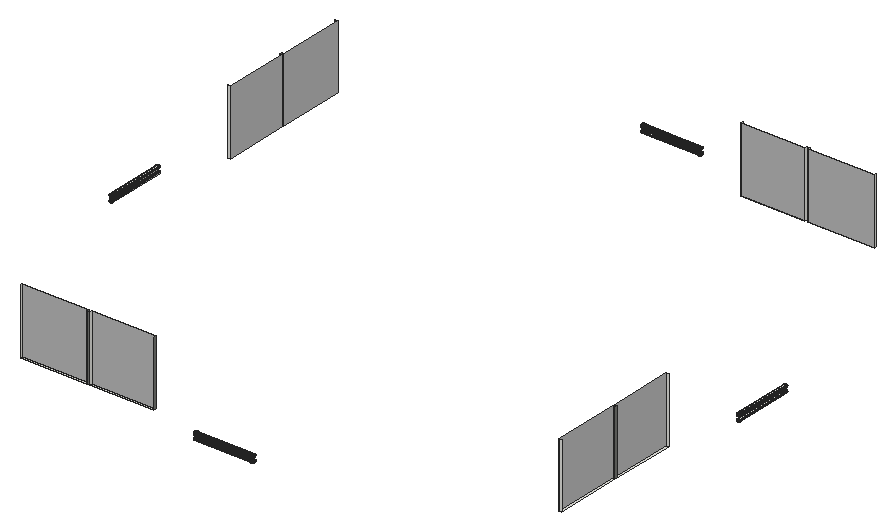
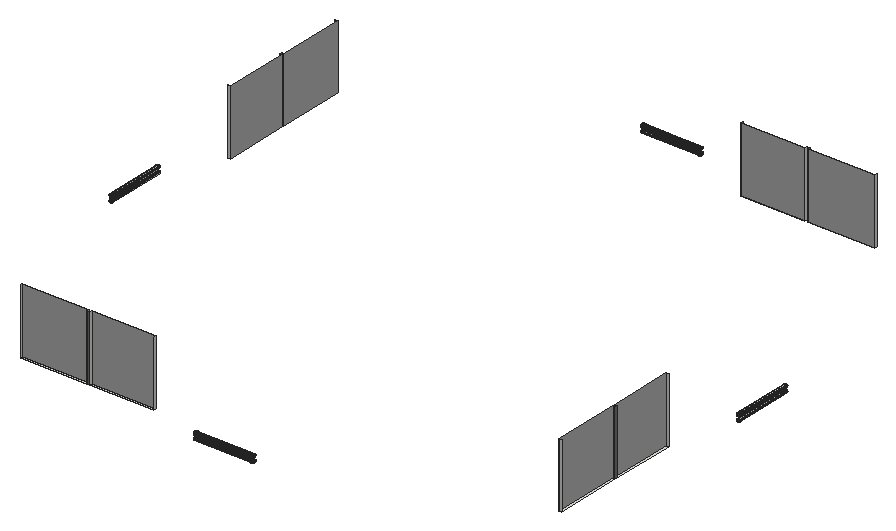
# SketchUp Ruby script. Lengths in inches.
U = 1.inch
M = Sketchup.active_model
def pt(a) = Geom::Point3d.new(a.map { |v| v * U })
def face(e, loops, mat)
  f = e.add_face(loops[0].map { |a| pt(a) })
  loops[1..].each { |l| e.add_face(l.map { |a| pt(a) }).erase! }
  f.material = f.back_material = mat if mat
  f
end
# faces: each face lists its corners as indices into pts; further lists are holes
def faces(e, pts, list, mat = nil) = list.each { |f| face(e, (f[0].is_a?(Array) ? f : [f]).map { |l| l.map { |i| pts[i] } }, mat) }
# xy, xz, yz: faces in a plane at the given z, y or x. An outline is a flat list of corners, or four numbers for a rectangle; further outlines are holes
def ring(l) = l.size == 4 ? [[l[0], l[1]], [l[2], l[1]], [l[2], l[3]], [l[0], l[3]]] : l.each_slice(2).to_a
def flat(e, list, mat, &to3) = list.each { |f| face(e, (f[0].is_a?(Array) ? f : [f]).map { |l| ring(l).map { |u, v| to3.(u, v) } }, mat) }
def xy(e, z, list, mat = nil) = flat(e, list, mat) { |x, y| [x, y, z] }
def xz(e, y, list, mat = nil) = flat(e, list, mat) { |x, z| [x, y, z] }
def yz(e, x, list, mat = nil) = flat(e, list, mat) { |y, z| [x, y, z] }
def lines(e, pts, list) = list.each { |a, b| e.add_line(pt(pts[a]), pt(pts[b])) }
# prism: a flat outline (further loops are holes) pulled along v
def prism(e, loops, v, mat = nil)
  f = face(e, loops, mat); d = Geom::Vector3d.new(v.map { |x| x * U })
  f.pushpull(f.normal.samedirection?(d) ? d.length : -d.length)
end
def box(e, o, s, mat = nil) = prism(e, [[o, [o[0] + s[0], o[1], o[2]], [o[0] + s[0], o[1] + s[1], o[2]], [o[0], o[1] + s[1], o[2]]]], [0, 0, s[2]], mat)
def at(x, y, z, deg = 0) = Geom::Transformation.translation(pt([x, y, z])) * Geom::Transformation.rotation(ORIGIN, Z_AXIS, deg.degrees)
def axes(o, x, y, z) = Geom::Transformation.new([*x, 0, *y, 0, *z, 0, *pt(o).to_a, 1])
def part(name) = M.definitions.add(name)
# library, detail: a bought-in or finely detailed component or shape, given as its bounding box
def library(name, o, s) = part(name).tap { |d| box(d.entities, o, s) }
def detail(e, o, s) = box(e.add_group.entities, o, s)
def put(e, d, t, mat = nil) = e.add_instance(d, t).tap { |i| i.material = mat if mat }
def group(e, t, mat = nil) = e.add_group.tap { |g| g.transformation = t; g.material = mat if mat }.entities
root = M.entities
M.materials.add("[Metal Seamed]").color = [118, 119, 115]
M.materials.add("[Mirror 01]").color = [185, 185, 185]
xy(root,899.76,[[312.65,102.8125,473.9375,108.8125],[479.9375,102.8125,635.22,108.8125],[1476,277.47,1482,438.75],[1476,444.75,1482,600.03],[138,949.59,144,1104.875],
  [138,1110.875,144,1272.16],[984.78,1440.8125,1140.0625,1446.8125],[1146.0625,1440.8125,1307.35,1446.8125]])
xz(root,102.8125,[[473.9375,899.76,479.9375,1056.625]],"[Metal Seamed]")
xz(root,108.8125,[[312.65,899.76,473.9375,1056.625],[479.9375,899.76,635.22,1056.625]],"[Mirror 01]")
xz(root,277.47,[[1476,899.76,1482,1056.625]])
xz(root,438.75,[[1476,899.76,1482,1056.625]])
xz(root,444.75,[[1476,899.76,1482,1056.625]])
xz(root,600.03,[[1476,899.76,1482,1056.625]])
xz(root,949.59,[[138,899.76,144,1056.625]])
xz(root,1104.875,[[138,899.76,144,1056.625]])
xz(root,1110.875,[[138,899.76,144,1056.625]])
xz(root,1272.16,[[138,899.76,144,1056.625]])
xz(root,1440.8125,[[984.78,899.76,1140.0625,1056.625],[1146.0625,899.76,1307.35,1056.625]],"[Mirror 01]")
xz(root,1446.8125,[[1140.0625,899.76,1146.0625,1056.625]],"[Metal Seamed]")
yz(root,138,[[1104.875,899.76,1110.875,1056.625]],"[Metal Seamed]")
yz(root,144,[[949.59,899.76,1104.875,1056.625],[1110.875,899.76,1272.16,1056.625]],"[Mirror 01]")
yz(root,312.65,[[102.8125,899.76,108.8125,1056.625]])
yz(root,473.9375,[[102.8125,899.76,108.8125,1056.625]],"[Metal Seamed]")
yz(root,479.9375,[[102.8125,899.76,108.8125,1056.625]])
yz(root,635.22,[[102.8125,899.76,108.8125,1056.625]],"[Metal Seamed]")
yz(root,984.78,[[1440.8125,899.76,1446.8125,1056.625]])
yz(root,1140.0625,[[1440.8125,899.76,1446.8125,1056.625]])
yz(root,1146.0625,[[1440.8125,899.76,1446.8125,1056.625]])
yz(root,1307.35,[[1440.8125,899.76,1446.8125,1056.625]])
yz(root,1476,[[277.47,899.76,438.75,1056.625],[444.75,899.76,600.03,1056.625]],"[Mirror 01]")
yz(root,1482,[[438.75,899.76,444.75,1056.625]],"[Metal Seamed]")
p = [[922.01,48.34,909.02],[922.01,47.38,909.14],[778.64,47.38,909.14],[778.64,48.34,909.02],[922.01,49.29,909.14],[778.64,49.29,909.14],
  [83.53,662.8,909.02],[82.57,662.8,909.14],[82.57,806.17,909.14],[83.53,806.17,909.02],[84.48,662.8,909.14],[84.48,806.17,909.14],
  [1535.52,886.83,909.14],[1536.47,886.83,909.02],[1536.47,743.45,909.02],[1535.52,743.45,909.14],[1537.43,886.83,909.14],[1537.43,743.45,909.14],
  [697.99,1500.33,909.14],[697.99,1501.28,909.02],[841.36,1501.28,909.02],[841.36,1500.33,909.14],[697.99,1502.24,909.14],[841.36,1502.24,909.14],
  [922.01,46.5,909.51],[778.64,46.5,909.51],[922.01,50.18,909.51],[778.64,50.18,909.51],[81.68,662.8,909.51],[81.68,806.17,909.51],
  [85.37,662.8,909.51],[85.37,806.17,909.51],[1534.63,886.83,909.51],[1534.63,743.45,909.51],[1538.32,886.83,909.51],[1538.32,743.45,909.51],
  [697.99,1499.44,909.51],[841.36,1499.44,909.51],[697.99,1503.13,909.51],[841.36,1503.13,909.51],[922.01,45.73,910.1],[778.64,45.73,910.1],
  [922.01,50.95,910.1],[778.64,50.95,910.1],[80.92,662.8,910.1],[80.92,806.17,910.1],[86.13,662.8,910.1],[86.13,806.17,910.1],
  [1533.87,886.83,910.1],[1533.87,743.45,910.1],[1539.08,886.83,910.1],[1539.08,743.45,910.1],[697.99,1498.68,910.1],[841.36,1498.68,910.1],
  [697.99,1503.89,910.1],[841.36,1503.89,910.1],[922.01,45.15,910.86],[778.64,45.15,910.86],[922.01,51.53,910.86],[778.64,51.53,910.86],
  [80.33,662.8,910.86],[80.33,806.17,910.86],[86.72,662.8,910.86],[86.72,806.17,910.86],[1533.28,886.83,910.86],[1533.28,743.45,910.86],
  [1539.67,886.83,910.86],[1539.67,743.45,910.86],[697.99,1498.09,910.86],[841.36,1498.09,910.86],[697.99,1504.48,910.86],[841.36,1504.48,910.86],
  [922.01,44.78,911.75],[778.64,44.78,911.75],[922.01,51.9,911.75],[778.64,51.9,911.75],[79.97,662.8,911.75],[79.97,806.17,911.75],
  [87.09,662.8,911.75],[87.09,806.17,911.75],[1532.91,886.83,911.75],[1532.91,743.45,911.75],[1540.03,886.83,911.75],[1540.03,743.45,911.75],
  [697.99,1497.72,911.75],[841.36,1497.72,911.75],[697.99,1504.85,911.75],[841.36,1504.85,911.75],[922.01,44.65,912.7],[778.64,44.65,912.7],
  [922.01,52.03,912.7],[778.64,52.03,912.7],[79.84,662.8,912.7],[79.84,806.17,912.7],[87.21,662.8,912.7],[87.21,806.17,912.7],
  [1532.79,886.83,912.7],[1532.79,743.45,912.7],[1540.16,886.83,912.7],[1540.16,743.45,912.7],[697.99,1497.6,912.7],[841.36,1497.6,912.7],
  [697.99,1504.97,912.7],[841.36,1504.97,912.7],[922.01,44.78,913.66],[778.64,44.78,913.66],[922.01,51.9,913.66],[778.64,51.9,913.66],
  [79.97,662.8,913.66],[79.97,806.17,913.66],[87.09,662.8,913.66],[87.09,806.17,913.66],[1532.91,886.83,913.66],[1532.91,743.45,913.66],
  [1540.03,886.83,913.66],[1540.03,743.45,913.66],[697.99,1497.72,913.66],[841.36,1497.72,913.66],[697.99,1504.85,913.66],[841.36,1504.85,913.66],
  [922.01,45.15,914.55],[778.64,45.15,914.55],[922.01,51.53,914.55],[778.64,51.53,914.55],[80.33,662.8,914.55],[80.33,806.17,914.55],
  [86.72,662.8,914.55],[86.72,806.17,914.55],[1533.28,886.83,914.55],[1533.28,743.45,914.55],[1539.67,886.83,914.55],[1539.67,743.45,914.55],
  [697.99,1498.09,914.55],[841.36,1498.09,914.55],[697.99,1504.48,914.55],[841.36,1504.48,914.55],[922.01,45.73,915.3125],[778.64,45.73,915.3125],
  [922.01,50.95,915.3125],[778.64,50.95,915.3125],[80.92,662.8,915.3125],[80.92,806.17,915.3125],[86.13,662.8,915.3125],[86.13,806.17,915.3125],
  [1533.87,886.83,915.3125],[1533.87,743.45,915.3125],[1539.08,886.83,915.3125],[1539.08,743.45,915.3125],[697.99,1498.68,915.3125],[841.36,1498.68,915.3125],
  [697.99,1503.89,915.3125],[841.36,1503.89,915.3125],[922.01,46.5,915.9],[778.64,46.5,915.9],[922.01,50.18,915.9],[778.64,50.18,915.9],
  [81.68,662.8,915.9],[81.68,806.17,915.9],[85.37,662.8,915.9],[85.37,806.17,915.9],[1534.63,886.83,915.9],[1534.63,743.45,915.9],
  [1538.32,886.83,915.9],[1538.32,743.45,915.9],[697.99,1499.44,915.9],[841.36,1499.44,915.9],[697.99,1503.13,915.9],[841.36,1503.13,915.9],
  [922.01,47.38,916.27],[778.64,47.38,916.27],[922.01,49.29,916.27],[778.64,49.29,916.27],[82.57,662.8,916.27],[82.57,806.17,916.27],
  [84.48,662.8,916.27],[84.48,806.17,916.27],[1535.52,886.83,916.27],[1535.52,743.45,916.27],[1537.43,886.83,916.27],[1537.43,743.45,916.27],
  [697.99,1500.33,916.27],[841.36,1500.33,916.27],[697.99,1502.24,916.27],[841.36,1502.24,916.27],[922.01,48.34,916.39],[778.64,48.34,916.39],
  [83.53,662.8,916.39],[83.53,806.17,916.39],[1536.47,886.83,916.39],[1536.47,743.45,916.39],[697.99,1501.28,916.39],[841.36,1501.28,916.39],
  [922.01,48.34,921.02],[922.01,47.38,921.14],[778.64,47.38,921.14],[778.64,48.34,921.02],[922.01,49.29,921.14],[778.64,49.29,921.14],
  [83.53,662.8,921.02],[82.57,662.8,921.14],[82.57,806.17,921.14],[83.53,806.17,921.02],[84.48,662.8,921.14],[84.48,806.17,921.14],
  [1535.52,886.83,921.14],[1536.47,886.83,921.02],[1536.47,743.45,921.02],[1535.52,743.45,921.14],[1537.43,886.83,921.14],[1537.43,743.45,921.14],
  [697.99,1500.33,921.14],[697.99,1501.28,921.02],[841.36,1501.28,921.02],[841.36,1500.33,921.14],[697.99,1502.24,921.14],[841.36,1502.24,921.14],
  [922.01,46.5,921.51],[778.64,46.5,921.51],[922.01,50.18,921.51],[778.64,50.18,921.51],[81.68,662.8,921.51],[81.68,806.17,921.51],
  [85.37,662.8,921.51],[85.37,806.17,921.51],[1534.63,886.83,921.51],[1534.63,743.45,921.51],[1538.32,886.83,921.51],[1538.32,743.45,921.51],
  [697.99,1499.44,921.51],[841.36,1499.44,921.51],[697.99,1503.13,921.51],[841.36,1503.13,921.51],[922.01,45.73,922.1],[778.64,45.73,922.1],
  [922.01,50.95,922.1],[778.64,50.95,922.1],[80.92,662.8,922.1],[80.92,806.17,922.1],[86.13,662.8,922.1],[86.13,806.17,922.1],
  [1533.87,886.83,922.1],[1533.87,743.45,922.1],[1539.08,886.83,922.1],[1539.08,743.45,922.1],[697.99,1498.68,922.1],[841.36,1498.68,922.1],
  [697.99,1503.89,922.1],[841.36,1503.89,922.1],[922.01,45.15,922.86],[778.64,45.15,922.86],[922.01,51.53,922.86],[778.64,51.53,922.86],
  [80.33,662.8,922.86],[80.33,806.17,922.86],[86.72,662.8,922.86],[86.72,806.17,922.86],[1533.28,886.83,922.86],[1533.28,743.45,922.86],
  [1539.67,886.83,922.86],[1539.67,743.45,922.86],[697.99,1498.09,922.86],[841.36,1498.09,922.86],[697.99,1504.48,922.86],[841.36,1504.48,922.86],
  [922.01,44.78,923.75],[778.64,44.78,923.75],[922.01,51.9,923.75],[778.64,51.9,923.75],[79.97,662.8,923.75],[79.97,806.17,923.75],
  [87.09,662.8,923.75],[87.09,806.17,923.75],[1532.91,886.83,923.75],[1532.91,743.45,923.75],[1540.03,886.83,923.75],[1540.03,743.45,923.75],
  [697.99,1497.72,923.75],[841.36,1497.72,923.75],[697.99,1504.85,923.75],[841.36,1504.85,923.75],[922.01,44.65,924.7],[778.64,44.65,924.7],
  [922.01,52.03,924.7],[778.64,52.03,924.7],[79.84,662.8,924.7],[79.84,806.17,924.7],[87.21,662.8,924.7],[87.21,806.17,924.7],
  [1532.79,886.83,924.7],[1532.79,743.45,924.7],[1540.16,886.83,924.7],[1540.16,743.45,924.7],[697.99,1497.6,924.7],[841.36,1497.6,924.7],
  [697.99,1504.97,924.7],[841.36,1504.97,924.7],[922.01,44.78,925.66],[778.64,44.78,925.66],[922.01,51.9,925.66],[778.64,51.9,925.66],
  [79.97,662.8,925.66],[79.97,806.17,925.66],[87.09,662.8,925.66],[87.09,806.17,925.66],[1532.91,886.83,925.66],[1532.91,743.45,925.66],
  [1540.03,886.83,925.66],[1540.03,743.45,925.66],[697.99,1497.72,925.66],[841.36,1497.72,925.66],[697.99,1504.85,925.66],[841.36,1504.85,925.66],
  [922.01,45.15,926.55],[778.64,45.15,926.55],[922.01,51.53,926.55],[778.64,51.53,926.55],[80.33,662.8,926.55],[80.33,806.17,926.55],
  [86.72,662.8,926.55],[86.72,806.17,926.55],[1533.28,886.83,926.55],[1533.28,743.45,926.55],[1539.67,886.83,926.55],[1539.67,743.45,926.55],
  [697.99,1498.09,926.55],[841.36,1498.09,926.55],[697.99,1504.48,926.55],[841.36,1504.48,926.55],[922.01,45.73,927.3125],[778.64,45.73,927.3125],
  [922.01,50.95,927.3125],[778.64,50.95,927.3125],[80.92,662.8,927.3125],[80.92,806.17,927.3125],[86.13,662.8,927.3125],[86.13,806.17,927.3125],
  [1533.87,886.83,927.3125],[1533.87,743.45,927.3125],[1539.08,886.83,927.3125],[1539.08,743.45,927.3125],[697.99,1498.68,927.3125],[841.36,1498.68,927.3125],
  [697.99,1503.89,927.3125],[841.36,1503.89,927.3125],[922.01,46.5,927.9],[778.64,46.5,927.9],[922.01,50.18,927.9],[778.64,50.18,927.9],
  [81.68,662.8,927.9],[81.68,806.17,927.9],[85.37,662.8,927.9],[85.37,806.17,927.9],[1534.63,886.83,927.9],[1534.63,743.45,927.9],
  [1538.32,886.83,927.9],[1538.32,743.45,927.9],[697.99,1499.44,927.9],[841.36,1499.44,927.9],[697.99,1503.13,927.9],[841.36,1503.13,927.9],
  [922.01,47.38,928.27],[778.64,47.38,928.27],[922.01,49.29,928.27],[778.64,49.29,928.27],[82.57,662.8,928.27],[82.57,806.17,928.27],
  [84.48,662.8,928.27],[84.48,806.17,928.27],[1535.52,886.83,928.27],[1535.52,743.45,928.27],[1537.43,886.83,928.27],[1537.43,743.45,928.27],
  [697.99,1500.33,928.27],[841.36,1500.33,928.27],[697.99,1502.24,928.27],[841.36,1502.24,928.27],[922.01,48.34,928.39],[778.64,48.34,928.39],
  [83.53,662.8,928.39],[83.53,806.17,928.39],[1536.47,886.83,928.39],[1536.47,743.45,928.39],[697.99,1501.28,928.39],[841.36,1501.28,928.39]]
faces(root,p,[[0,1,2,3],[4,0,3,5],[6,7,8,9],[10,6,9,11],[12,13,14,15],[13,16,17,14],[18,19,20,21],[19,22,23,20],
  [1,24,25,2],[26,4,5,27],[7,28,29,8],[30,10,11,31],[32,12,15,33],[16,34,35,17],[36,18,21,37],[22,38,39,23],
  [24,40,41,25],[42,26,27,43],[28,44,45,29],[46,30,31,47],[48,32,33,49],[34,50,51,35],[52,36,37,53],[38,54,55,39],
  [40,56,57,41],[58,42,43,59],[44,60,61,45],[62,46,47,63],[64,48,49,65],[50,66,67,51],[68,52,53,69],[54,70,71,55],
  [56,72,73,57],[74,58,59,75],[60,76,77,61],[78,62,63,79],[80,64,65,81],[66,82,83,67],[84,68,69,85],[70,86,87,71],
  [72,88,89,73],[90,74,75,91],[76,92,93,77],[94,78,79,95],[96,80,81,97],[82,98,99,83],[100,84,85,101],[86,102,103,87],
  [88,104,105,89],[106,90,91,107],[92,108,109,93],[110,94,95,111],[112,96,97,113],[98,114,115,99],[116,100,101,117],[102,118,119,103],
  [104,120,121,105],[122,106,107,123],[108,124,125,109],[126,110,111,127],[128,112,113,129],[114,130,131,115],[132,116,117,133],[118,134,135,119],
  [120,136,137,121],[138,122,123,139],[124,140,141,125],[142,126,127,143],[144,128,129,145],[130,146,147,131],[148,132,133,149],[134,150,151,135],
  [136,152,153,137],[154,138,139,155],[140,156,157,141],[158,142,143,159],[160,144,145,161],[146,162,163,147],[164,148,149,165],[150,166,167,151],
  [152,168,169,153],[170,154,155,171],[156,172,173,157],[174,158,159,175],[176,160,161,177],[162,178,179,163],[180,164,165,181],[166,182,183,167],
  [168,184,185,169],[184,170,171,185],[172,186,187,173],[186,174,175,187],[188,176,177,189],[178,188,189,179],[190,180,181,191],[182,190,191,183],
  [192,193,194,195],[196,192,195,197],[198,199,200,201],[202,198,201,203],[204,205,206,207],[205,208,209,206],[210,211,212,213],[211,214,215,212],
  [193,216,217,194],[218,196,197,219],[199,220,221,200],[222,202,203,223],[224,204,207,225],[208,226,227,209],[228,210,213,229],[214,230,231,215],
  [216,232,233,217],[234,218,219,235],[220,236,237,221],[238,222,223,239],[240,224,225,241],[226,242,243,227],[244,228,229,245],[230,246,247,231],
  [232,248,249,233],[250,234,235,251],[236,252,253,237],[254,238,239,255],[256,240,241,257],[242,258,259,243],[260,244,245,261],[246,262,263,247],
  [248,264,265,249],[266,250,251,267],[252,268,269,253],[270,254,255,271],[272,256,257,273],[258,274,275,259],[276,260,261,277],[262,278,279,263],
  [264,280,281,265],[282,266,267,283],[268,284,285,269],[286,270,271,287],[288,272,273,289],[274,290,291,275],[292,276,277,293],[278,294,295,279],
  [280,296,297,281],[298,282,283,299],[284,300,301,285],[302,286,287,303],[304,288,289,305],[290,306,307,291],[308,292,293,309],[294,310,311,295],
  [296,312,313,297],[314,298,299,315],[300,316,317,301],[318,302,303,319],[320,304,305,321],[306,322,323,307],[324,308,309,325],[310,326,327,311],
  [312,328,329,313],[330,314,315,331],[316,332,333,317],[334,318,319,335],[336,320,321,337],[322,338,339,323],[340,324,325,341],[326,342,343,327],
  [328,344,345,329],[346,330,331,347],[332,348,349,333],[350,334,335,351],[352,336,337,353],[338,354,355,339],[356,340,341,357],[342,358,359,343],
  [344,360,361,345],[362,346,347,363],[348,364,365,349],[366,350,351,367],[368,352,353,369],[354,370,371,355],[372,356,357,373],[358,374,375,359],
  [360,376,377,361],[376,362,363,377],[364,378,379,365],[378,366,367,379],[380,368,369,381],[370,380,381,371],[382,372,373,383],[374,382,383,375]])
